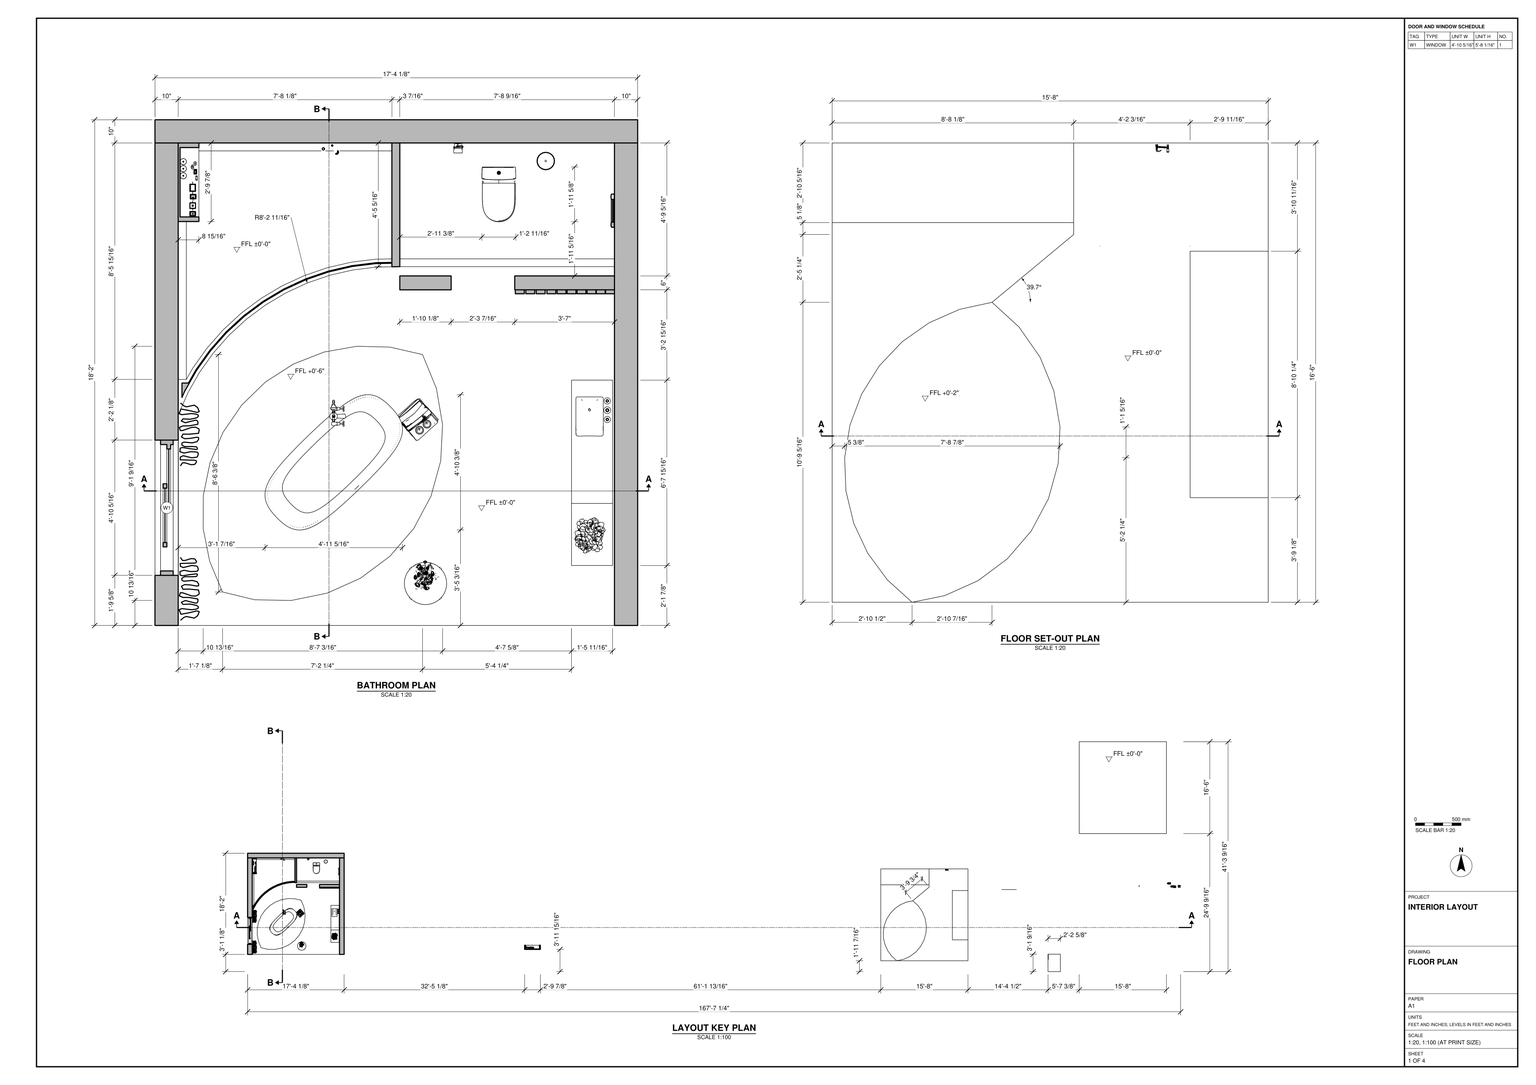
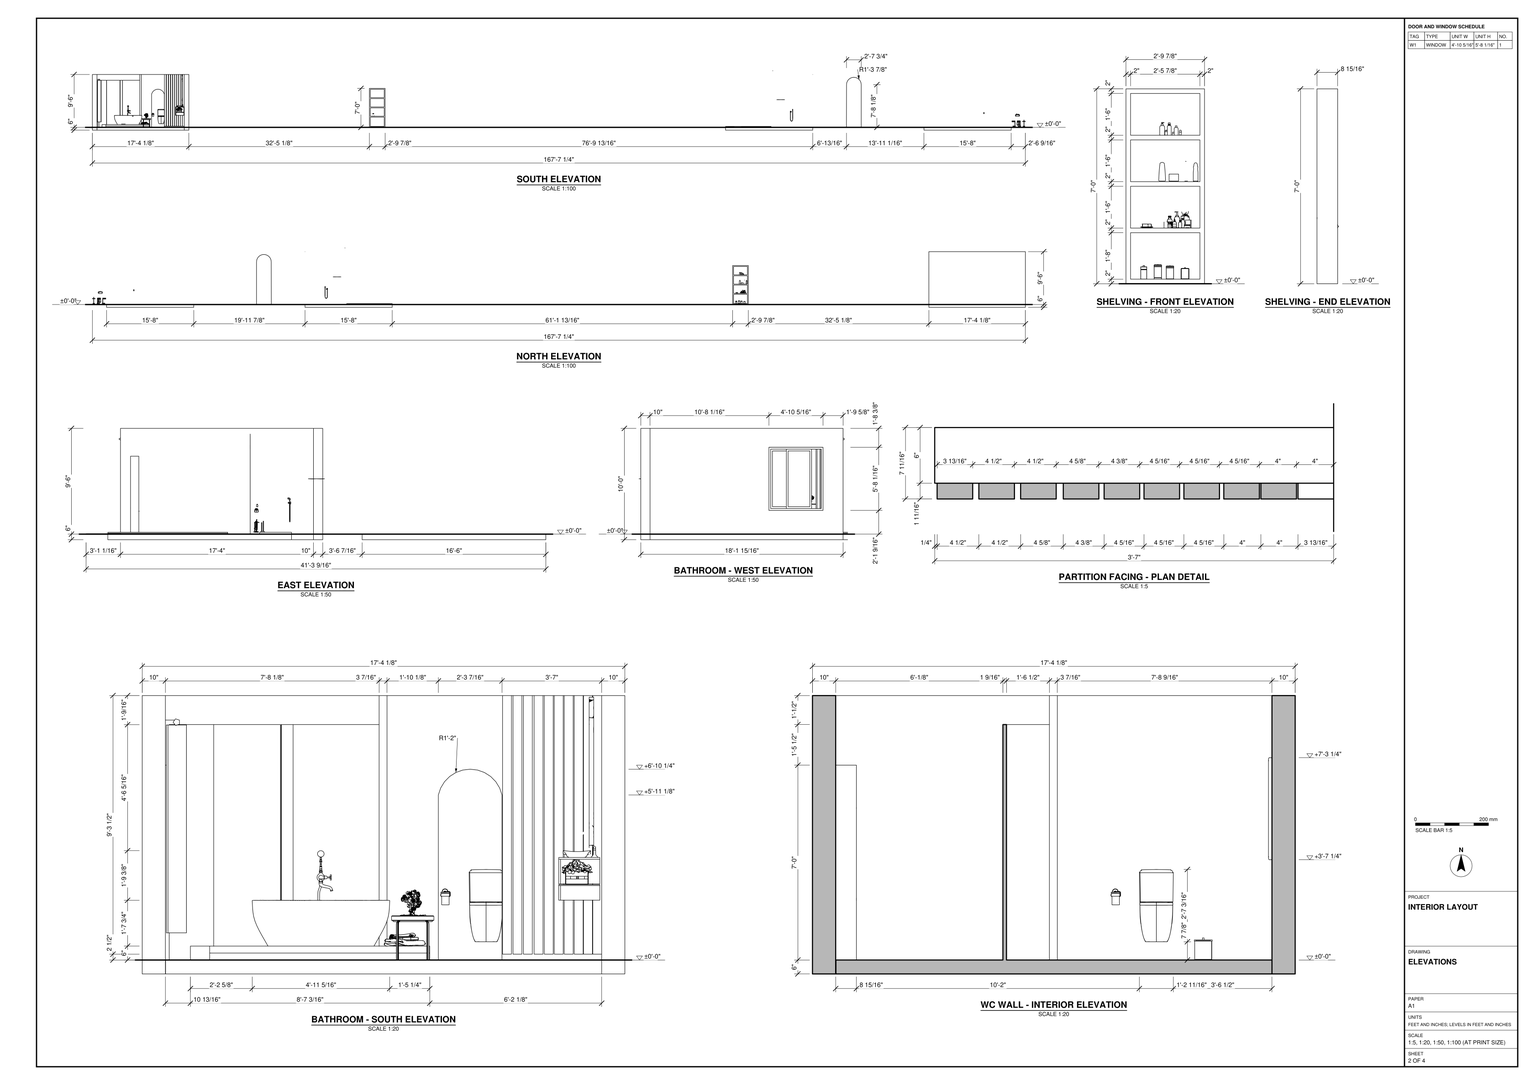
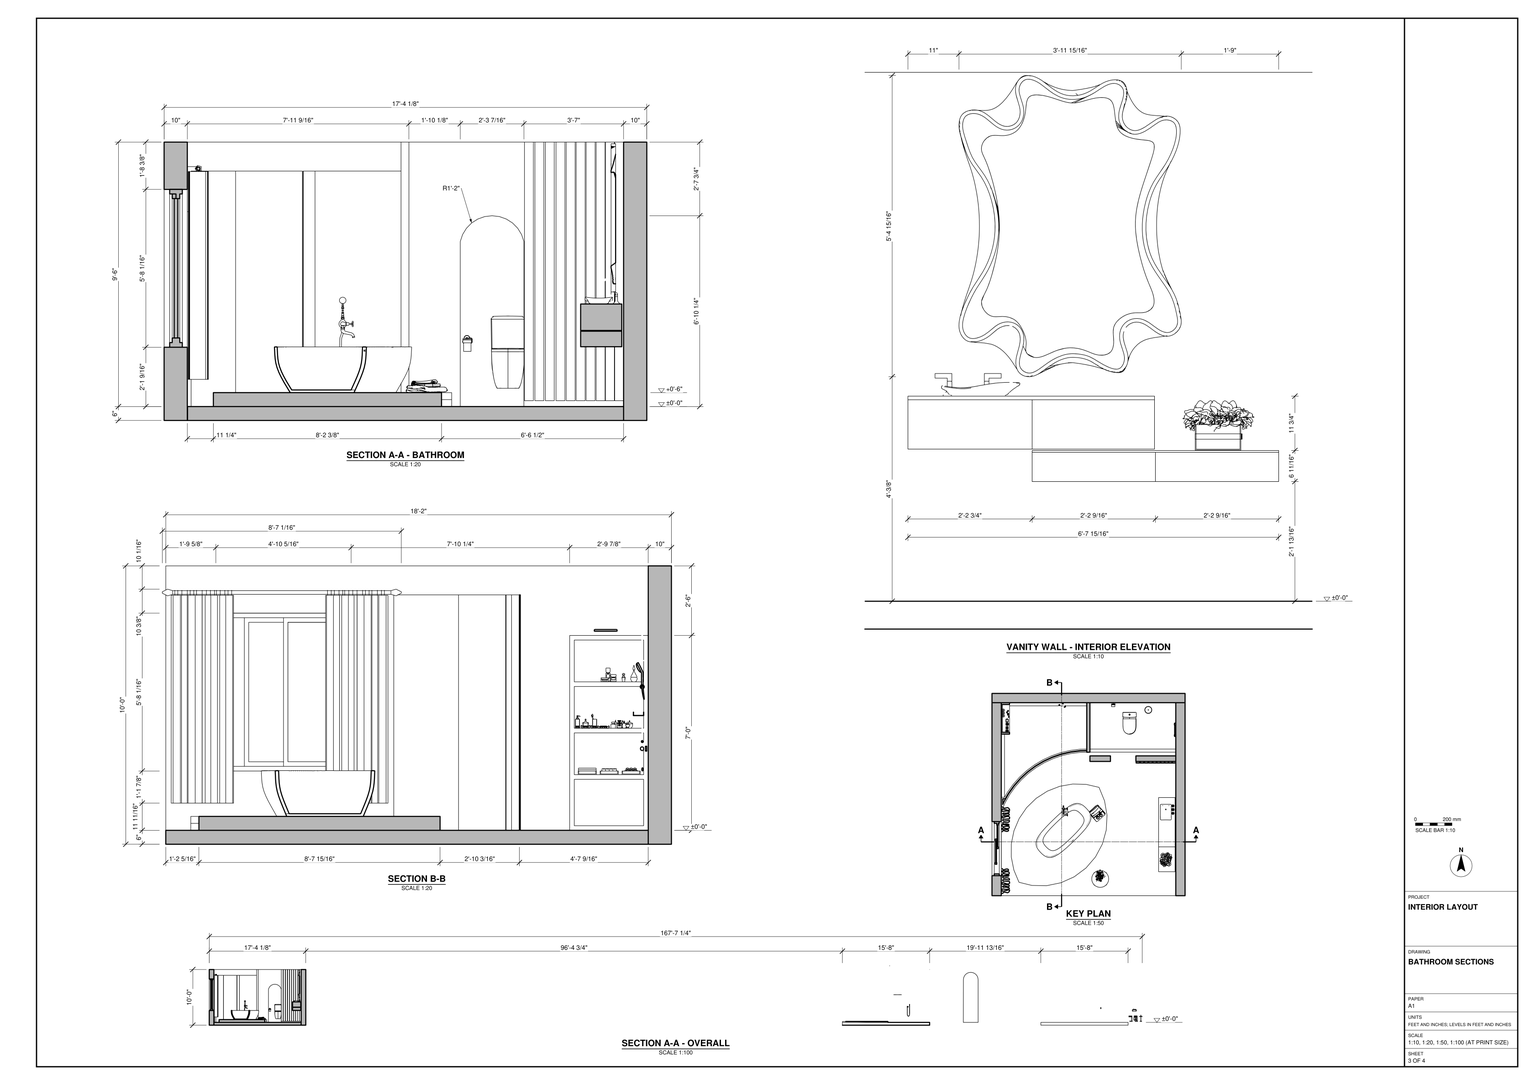
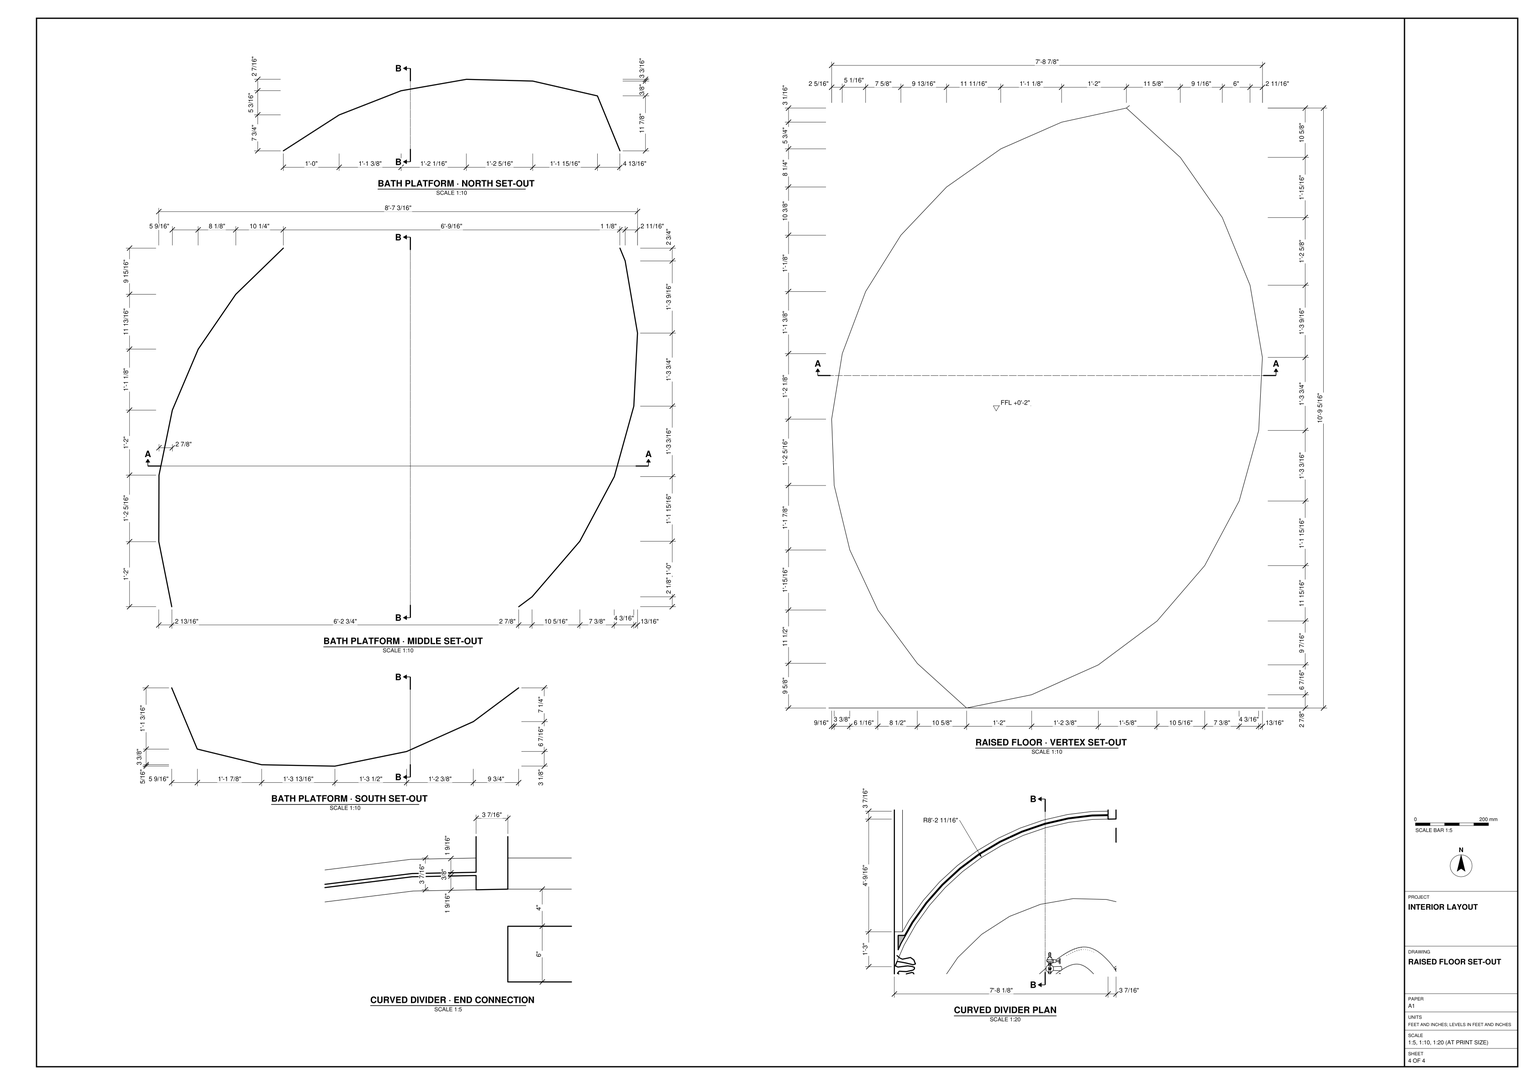
Work in feet and inches in SketchUp using task_files/diagram_01.pdf. Use the layout key plan to position the fitted bathroom at the left and the separate shelving, floor set-out pieces and fittings to its right. Keep the spaces between them as drawn. The complete layout is 167'-7 1/4" along X, 41'-3 9/16" along Y and 10'-0" high. Use ±0'-0" as the single storey datum.

Build the bathroom shell to its own plan dimensions of 17'-4 1/8" by 18'-2", with the floor slab, 10" perimeter walls and internal partitions at their drawn thicknesses. Form the framed west window above its sill. Set the freestanding tub diagonally on the rounded platform, with the tub filler and small table beside it. Follow the curve separating the shower area from the bath, and model the rear toilet compartment with its round-headed opening and adjacent slatted facing.

Use the interior elevations to build the stepped, wall-hung vanity with its basin and mirror, and the open shelving with its horizontal compartments. Reproduce the floor outlines and changes in height shown in the plan and sections, distinguishing the platform in the bathroom from the separate floor set-out. Decor and loose items, including curtains, plants and toiletries, may be any suitable library components.

Keep shell elements and each furniture or joinery piece in separate groups or components, and use components for repeated parts. Save one SketchUp model as output_files/bathroom_interior_and_its_separate_set_out_elements.skp.

# SketchUp Ruby script. Lengths in inches.
U = 1.inch
M = Sketchup.active_model
def pt(a) = Geom::Point3d.new(a.map { |v| v * U })
def face(e, loops, mat)
  f = e.add_face(loops[0].map { |a| pt(a) })
  loops[1..].each { |l| e.add_face(l.map { |a| pt(a) }).erase! }
  f.material = f.back_material = mat if mat
  f
end
# faces: each face lists its corners as indices into pts; further lists are holes
def faces(e, pts, list, mat = nil) = list.each { |f| face(e, (f[0].is_a?(Array) ? f : [f]).map { |l| l.map { |i| pts[i] } }, mat) }
# xy, xz, yz: faces in a plane at the given z, y or x. An outline is a flat list of corners, or four numbers for a rectangle; further outlines are holes
def ring(l) = l.size == 4 ? [[l[0], l[1]], [l[2], l[1]], [l[2], l[3]], [l[0], l[3]]] : l.each_slice(2).to_a
def flat(e, list, mat, &to3) = list.each { |f| face(e, (f[0].is_a?(Array) ? f : [f]).map { |l| ring(l).map { |u, v| to3.(u, v) } }, mat) }
def xy(e, z, list, mat = nil) = flat(e, list, mat) { |x, y| [x, y, z] }
def xz(e, y, list, mat = nil) = flat(e, list, mat) { |x, z| [x, y, z] }
def yz(e, x, list, mat = nil) = flat(e, list, mat) { |y, z| [x, y, z] }
def lines(e, pts, list) = list.each { |a, b| e.add_line(pt(pts[a]), pt(pts[b])) }
# prism: a flat outline (further loops are holes) pulled along v
def prism(e, loops, v, mat = nil)
  f = face(e, loops, mat); d = Geom::Vector3d.new(v.map { |x| x * U })
  f.pushpull(f.normal.samedirection?(d) ? d.length : -d.length)
end
def box(e, o, s, mat = nil) = prism(e, [[o, [o[0] + s[0], o[1], o[2]], [o[0] + s[0], o[1] + s[1], o[2]], [o[0], o[1] + s[1], o[2]]]], [0, 0, s[2]], mat)
def at(x, y, z, deg = 0) = Geom::Transformation.translation(pt([x, y, z])) * Geom::Transformation.rotation(ORIGIN, Z_AXIS, deg.degrees)
def axes(o, x, y, z) = Geom::Transformation.new([*x, 0, *y, 0, *z, 0, *pt(o).to_a, 1])
def part(name) = M.definitions.add(name)
# library, detail: a bought-in or finely detailed component or shape, given as its bounding box
def library(name, o, s) = part(name).tap { |d| box(d.entities, o, s) }
def detail(e, o, s) = box(e.add_group.entities, o, s)
def put(e, d, t, mat = nil) = e.add_instance(d, t).tap { |i| i.material = mat if mat }
def group(e, t, mat = nil) = e.add_group.tap { |g| g.transformation = t; g.material = mat if mat }.entities
root = M.entities
M.materials.add("[Color A01]").color = [255, 204, 204]
M.materials.add("[Color A02]").color = [255, 153, 153]
M.materials.add("[Color B01]").color = [207, 197, 189]
M.materials.add("[Translucent Glass Blue]").color = [100, 149, 237]
M.materials["[Translucent Glass Blue]"].alpha = 0.5
c1 = library("bath+tub",[751.79,-1619.37,0],[68.45,31.82,19.75])
c2 = library("Inodoro ROCA Meridian-N compact",[-14.68,0,0],[14.68,23.62,31.16])
c3 = library("77732 KARE Mirror Drops Oval 14x25cm (Spiegel Drops Oval 14x",[-0.49,-2.625,-0.01],[0.98,5.28,9.78])
c4 = library("Group\#95",[-126.0625,56.51,376.27],[112.05,106.35,108.99])
c5 = library("Group\#96",[-107.16,-137.18,245.54],[76.51,112.05,84.97])
c6 = library("Group\#98",[134.07,-35.59,197.42],[66.93,108.39,101.45])
c7 = library("Group\#99",[44.02,93.6,218.34],[115.22,101.76,105.18])
c8 = library("Group\#100",[-19.56,232.65,283.18],[66.82,42.19,66.65])
c9 = library("Group\#101",[-53.74,7.67,120.98],[106.95,236.74,251.98])
c10 = library("Group\#102",[-49.75,139.84,314.95],[22.11,22.61,22.06])
c11 = library("Group\#103",[-56.625,3.66,294.95],[88.3,152.82,59.14])
c12 = library("Group\#107",[-100.48,19.53,147.87],[113.05,111.28,101.19])
c13 = library("Group\#108",[-54.85,-171.1875,247.55],[90.72,132.3,71.07])
c14 = library("Group\#111",[-161.51,-101.97,314.73],[172.81,108.71,69.27])
c15 = library("Group\#113",[70.77,-125.64,148.84],[102.7,108.07,96.82])
c16 = library("Group\#114",[-28.1,-125.85,106.48],[194.72,128.52,261.01])
c17 = library("Group\#115",[-14.51,-199.73,94.2],[105.22,97.74,77.03])
c18 = library("Group\#116",[-24.89,-182.93,111.64],[113.72,173.94,173.74])
c19 = library("Group\#117",[-7.79,-309.02,238.22],[108.5,93.72,102.44])
c20 = library("Group\#118",[2.57,-271.06,187.04],[93.4,209.89,191.26])
c21 = library("Group\#119",[-21.74,-164.88,146.75],[158.66,158.69,243.45])
c22 = library("Group\#120",[51.13,-202.98,245.86],[103.83,96.91,120.11])
c23 = library("Group\#121",[111.16,-90.29,303.89],[49.95,90,76.18])
c24 = library("Group\#122",[47.44,-177.11,343.1],[125.1,149.08,142.01])
c25 = library("Group\#123",[-80.82,10.33,268.03],[91.87,74,84.35])
c26 = library("Group\#124",[-75.58,-212.0625,396.64],[87.14,69.73,75.82])
c27 = library("Group\#125",[-86.85,-171.15,214.86],[148.39,157.28,240.38])
c28 = library("Group\#126",[-191.98,-250.23,297.57],[97.9,89.36,114.5])
c29 = library("Group\#127",[-192.01,-26.24,304.89],[187.25,107.21,53.21])
c30 = library("Group\#128",[-210.125,-102.4375,276.88],[51.54,90.91,87.28])
c31 = library("Group\#129",[-168.05,-105.3,214.4],[173.05,109.74,165.51])
c32 = library("Group\#130",[-147.09,-43.87,347.03],[63.89,87.81,80.15])
c33 = library("Group\#131",[-110.02,-64.26,144.44],[128.07,118.55,275.77])
c34 = library("Group\#132",[-124.14,3.49,256.66],[120.45,70.64,46.18])
c35 = library("Group\#133",[-118.71,-26.72,138.49],[113,166.64,338.37])
c36 = library("Group\#134",[-159.97,129.63,257.39],[89.36,80.73,106.4])
c37 = library("Group\#135",[-136.13,-14.65,175.64],[147.69,202.17,192.49])
c38 = library("Group\#136",[-5.59,-15.12,374.79],[85.57,86.81,59.51])
c39 = library("Group\#137",[-37.32,-33.18,117.69],[148.47,104.95,286.6])
c40 = library("Group\#138",[-6.61,93.85,461.94],[98.68,62.42,49.38])
c41 = library("Group\#139",[-20.13,5.57,225.44],[155.68,162.88,267.12])
c42 = library("Group\#140",[-80.73,-182.31,261.98],[90.74,132.73,71.97])
c43 = library("Group\#141",[-75.53,-189.01,309.71],[68.94,147.24,88.69])
c44 = library("Group\#142",[-39.42,-209.09,286.91],[66.94,168.34,116.98])
c45 = library("Group\#143",[-81.93,-128.91,211.16],[107.53,90.8,94.63])
c46 = library("Group\#144",[-21.54,14.12,313.18],[84.79,137.02,109.55])
c47 = library("Group\#145",[-45.26,-82.43,273.6875],[73.19,105.45,181.93])
c48 = library("Group\#146",[-10.36,3.03,272.26],[79.07,139.88,53.94])
c49 = library("Group\#147",[24.16,-5.45,296.62],[84.08,128.04,53.21])
c50 = library("Group\#148",[-40.71,1.11,275.78],[91.4,147.63,75.64])
c51 = library("Group\#149",[1.16,-23.73,246.66],[101.27,126.17,86.62])
c52 = library("Group\#150",[-53.8125,-212.33,295.34],[68.49,139.76,73.67])
c53 = library("Group\#151",[-94.36,-157.31,255.2],[101.84,115.08,71.07])
c54 = library("Group\#152",[-39.88,-92.9,113.08],[80.99,54.06,154.09])
c55 = library("Group\#153",[-59.78,14.09,300.39],[101.06,171.37,85.05])
c56 = library("Group\#154",[-39.96,0.65,262.91],[71.32,151.8,74.06])
c57 = library("Group\#155",[-161.17,-232.45,32.75],[152.53,236.06,399.97])
c58 = library("Group\#156",[6.78,-176.96,61.53],[128.84,205.63,400.02])
c59 = library("Group\#157",[-1.6875,-94.42,75.86],[134.92,113.41,305.11])
c60 = library("Group\#158",[-60.84,-159.99,77.97],[92.87,130.98,190.36])
c61 = library("Group\#159",[-62.72,-147.62,57.55],[93.45,86.61,60.22])
c62 = library("Group\#160",[-84.97,-34.6875,78.05],[116.39,151.55,263.18])
c63 = library("Group\#161",[-32.97,-25.89,74.09],[206.79,187.79,274.23])
c64 = library("Group\#162",[-54.58,-83.54,30.99],[209.74,138.81,269.85])
c65 = library("Group\#163",[-44.59,-71.91,-0.375],[108.06,108.06,265.92])
c66 = library("Group\#164",[-41.5,-68.73,2.45],[101.74,101.7,171.82])
c67 = library("Group\#165",[-41.09,-203.71,-2.45],[72.23,68.1,8.96])
c68 = library("Group\#166",[-72.08,-328.41,-0.84],[78.06,90.26,14.33])
c69 = library("Group\#167",[-38.17,-273.34,-0.36],[93.61,85.68,37.86])
c70 = library("Group\#168",[-44.12,-281.8,-0.32],[111.26,106.83,75.57])
c71 = library("Group\#169",[79.9,102.31,0.95],[37.36,48.66,9.9])
c72 = library("Group\#170",[56.48,112.77,1.08],[48.06,25.98,13.89])
c73 = library("Group\#171",[72.44,-147.39,-0.42],[23.31,46.98,9.15])
c74 = library("Group\#172",[210.7,-108.99,0.28],[36.24,50.48,9.9])
c75 = library("Group\#173",[220.9,-124.54,1.08],[13.77,52.12,13.89])
c76 = library("Group\#174",[167.26,-103.49,-0.7],[57.68,26.7,10.44])
c77 = library("Group\#175",[142.48,-79.67,1],[43.05,39.63,15.57])
c78 = library("Group\#176",[248.67,-54.61,-0.08],[36.39,42.46,17.38])
c79 = library("Group\#177",[193.58,-33.21,-1.68],[36.48,42.01,10.95])
c80 = library("Group\#179",[210.09,-29.63,-0.2],[39.11,52.61,14.77])
c81 = library("Group\#180",[-209.51,-88.09,-0.09],[13.54,51.1,15.8])
c82 = library("Group\#181",[-54.86,-136.11,-1.68],[49.86,19.04,10.95])
c83 = library("Group\#183",[-122.87,-196.19,0.47],[48.06,25.97,13.89])
c84 = library("Group\#184",[-150.12,-240.625,-0.4],[11.63,50.1,24.95])
c85 = library("Group\#185",[-116.51,-130.79,0.39],[14.38,57.14,15.57])
c86 = library("Group\#186",[-182.24,-139.72,-0.13],[56.75,40.03,14.2])
c87 = library("Group\#188",[-207.67,30.42,-0.9],[25.63,50.27,12.3])
c88 = library("Group\#189",[-172.77,40.41,-0.51],[21.75,45.25,16.32])
c89 = library("Group\#190",[-180.55,189.74,-0.03],[49.43,32.8,20.41])
c90 = library("Group\#191",[101.2,192.9375,0.85],[30.56,51.07,18.99])
c91 = library("Group\#192",[-229.59,150.48,-0.31],[49.39,18.82,9.67])
c92 = library("Group\#193",[-112.85,170.09,0.27],[33.5,38.18,12.42])
c93 = library("Group\#194",[21.88,30.1,1.13],[19.79,43.29,9.19])
c94 = library("Group\#195",[-79.42,-90.58,1.23],[27.88,43.88,12.3])
c95 = library("Group\#196",[-127.08,-286.71,-0.14],[33.47,50.32,11.84])
c96 = library("Group\#197",[-197.39,99.82,-0.47],[43.11,37.62,15.6])
c97 = library("Group\#199",[-27.41,-124.52,-0.78],[20.93,47.82,9.14])
c98 = library("Group\#200",[26.33,74.99,1.28],[53.38,19.42,14.98])
c99 = library("Group\#201",[10.45,76.82,0.07],[28.28,56.98,13.56])
c100 = library("Group\#202",[-25.11,33.28,1.57],[29.78,42.64,16.1])
c101 = library("Group\#203",[-39.97,68.22,-0.03],[38.63,48.26,26.54])
c102 = library("Group\#204",[164.13,106.84,0.59],[27.38,60.49,14.93])
c103 = library("Group\#205",[-130.15,4.41,-0.48],[48.46,51.92,11.15])
c104 = library("Group\#206",[-189.65,-8.38,0.66],[48.33,31.91,9.88])
c105 = library("Group\#207",[-141.44,-113.37,0.3],[20.53,61.5,14.1])
c106 = library("Group\#208",[-0.86,206.91,0.32],[47.68,39.6,11.54])
c107 = library("Group\#209",[-44.14,156.6,-1.15],[45.04,36.23,10.11])
c108 = library("Group\#210",[20.74,116.14,-1.25],[18.97,49.31,11.1])
c109 = library("Group\#211",[82.73,35.89,0.36],[52.87,25.75,10.37])
c110 = library("Group\#212",[-127.82,-180.79,-0.25],[32.53,51.61,10.43])
c111 = library("Group\#213",[-174.32,-293.63,-0.39],[47.63,19.69,18.01])
c112 = library("Group\#214",[-99.45,-206.66,0.34],[37.36,48.66,9.91])
c113 = library("Group\#215",[-200.03,-84.69,-0.65],[59.14,46.37,12.98])
c114 = library("Group\#216",[-110.43,96.29,-0.82],[45.84,41.98,9.65])
c115 = library("Group\#217",[-81.31,-44.23,0.64],[38.81,47.66,17.39])
c116 = library("Group\#220",[162.0625,4.5,-0.42],[38.34,35.6875,9.15])
c117 = part("flower vase")
p = [[0,0,0],[1,0,0],[1,1,0]]
lines(c117.entities,p,[[0,1],[1,2],[2,0]])
put(c117.entities,c4,at(0,0,0))
put(c117.entities,c5,at(0,0,0))
put(c117.entities,c6,at(0,0,0))
put(c117.entities,c7,at(0,0,0))
put(c117.entities,c8,at(0,0,0))
put(c117.entities,c9,at(0,0,0))
put(c117.entities,c10,at(0,0,0))
put(c117.entities,c11,at(0,0,0))
put(c117.entities,c12,at(0,0,0))
put(c117.entities,c13,at(0,0,0))
put(c117.entities,c14,at(0,0,0))
put(c117.entities,c15,at(0,0,0))
put(c117.entities,c16,at(0,0,0))
put(c117.entities,c17,at(0,0,0))
put(c117.entities,c18,at(0,0,0))
put(c117.entities,c19,at(0,0,0))
put(c117.entities,c20,at(0,0,0))
put(c117.entities,c21,at(0,0,0))
put(c117.entities,c22,at(0,0,0))
put(c117.entities,c23,at(0,0,0))
put(c117.entities,c24,at(0,0,0))
put(c117.entities,c25,at(0,0,0))
put(c117.entities,c26,at(0,0,0))
put(c117.entities,c27,at(0,0,0))
put(c117.entities,c28,at(0,0,0))
put(c117.entities,c29,at(0,0,0))
put(c117.entities,c30,at(0,0,0))
put(c117.entities,c31,at(0,0,0))
put(c117.entities,c32,at(0,0,0))
put(c117.entities,c33,at(0,0,0))
put(c117.entities,c34,at(0,0,0))
put(c117.entities,c35,at(0,0,0))
put(c117.entities,c36,at(0,0,0))
put(c117.entities,c37,at(0,0,0))
put(c117.entities,c38,at(0,0,0))
put(c117.entities,c39,at(0,0,0))
put(c117.entities,c40,at(0,0,0))
put(c117.entities,c41,at(0,0,0))
put(c117.entities,c42,at(0,0,0))
put(c117.entities,c43,at(0,0,0))
put(c117.entities,c44,at(0,0,0))
put(c117.entities,c45,at(0,0,0))
put(c117.entities,c46,at(0,0,0))
put(c117.entities,c47,at(0,0,0))
put(c117.entities,c48,at(0,0,0))
put(c117.entities,c49,at(0,0,0))
put(c117.entities,c50,at(0,0,0))
put(c117.entities,c51,at(0,0,0))
put(c117.entities,c52,at(0,0,0))
put(c117.entities,c53,at(0,0,0))
put(c117.entities,c54,at(0,0,0))
put(c117.entities,c55,at(0,0,0))
put(c117.entities,c56,at(0,0,0))
put(c117.entities,c57,at(0,0,0))
put(c117.entities,c58,at(0,0,0))
put(c117.entities,c59,at(0,0,0))
put(c117.entities,c60,at(0,0,0))
put(c117.entities,c61,at(0,0,0))
put(c117.entities,c62,at(0,0,0))
put(c117.entities,c63,at(0,0,0))
put(c117.entities,c64,at(0,0,0))
put(c117.entities,c65,at(0,0,0))
put(c117.entities,c66,at(0,0,0))
put(c117.entities,c67,at(0,0,0))
put(c117.entities,c68,at(0,0,0))
put(c117.entities,c69,at(0,0,0))
put(c117.entities,c70,at(0,0,0))
put(c117.entities,c71,at(0,0,0))
put(c117.entities,c72,at(0,0,0))
put(c117.entities,c73,at(0,0,0))
put(c117.entities,c74,at(0,0,0))
put(c117.entities,c75,at(0,0,0))
put(c117.entities,c76,at(0,0,0))
put(c117.entities,c77,at(0,0,0))
put(c117.entities,c78,at(0,0,0))
put(c117.entities,c79,at(0,0,0))
g1 = group(c117.entities,at(0,0,0))
detail(g1,[-125.92,-57.19,0],[29.51,42.66,5.27])
put(c117.entities,c80,at(0,0,0))
put(c117.entities,c81,at(0,0,0))
put(c117.entities,c82,at(0,0,0))
g2 = group(c117.entities,at(0,0,0))
detail(g2,[-72.81,-133.6875,-0.86],[7.83,54.32,7.6])
put(c117.entities,c83,at(0,0,0))
put(c117.entities,c84,at(0,0,0))
put(c117.entities,c85,at(0,0,0))
put(c117.entities,c86,at(0,0,0))
g3 = group(c117.entities,at(0,0,0))
detail(g3,[-128.51,132.875,-0.52],[47.95,16.21,8.19])
put(c117.entities,c87,at(0,0,0))
put(c117.entities,c88,at(0,0,0))
put(c117.entities,c89,at(0,0,0))
put(c117.entities,c90,at(0,0,0))
put(c117.entities,c91,at(0,0,0))
put(c117.entities,c92,at(0,0,0))
put(c117.entities,c93,at(0,0,0))
put(c117.entities,c94,at(0,0,0))
put(c117.entities,c95,at(0,0,0))
put(c117.entities,c96,at(0,0,0))
g4 = group(c117.entities,at(0,0,0))
p = [[-27.64,62.67,3.44],[-15.71,68.26,1.48],[-15.66,71.65,0.62],[-21.57,68.97,2.31],[-13.17,69.58,2.55],[-36.26,54.21,1.61],
  [-31.87,53.51,1.99],[-33.2,58.14,1.29],[-31.35,61.65,2.625],[-15.72,67.39,3.15],[-44.8,46.65,5.28],[-47.1,43.13,7.82],
  [-28.86,58.34,3.52],[-29.19,65.03,3.4],[-25.6,67.375,2.31],[-22.51,63.64,4.02],[-26.57,61.08,4.77],[-48.1,43.35,7.41],
  [-48.18,44.3,7.4]]
faces(g4,p,[[0,1,2],[3,0,2],[2,1,4],[5,6,7],[0,7,6],[0,8,7],[0,9,1],[10,6,5],
  [10,11,6],[0,6,12],[13,0,14],[0,3,14],[0,13,8],[0,15,9],[12,16,0],[0,16,15],
  [17,11,10],[10,18,17]])
put(c117.entities,c97,at(0,0,0))
put(c117.entities,c98,at(0,0,0))
put(c117.entities,c99,at(0,0,0))
put(c117.entities,c100,at(0,0,0))
put(c117.entities,c101,at(0,0,0))
put(c117.entities,c102,at(0,0,0))
put(c117.entities,c103,at(0,0,0))
put(c117.entities,c104,at(0,0,0))
put(c117.entities,c105,at(0,0,0))
put(c117.entities,c106,at(0,0,0))
put(c117.entities,c107,at(0,0,0))
put(c117.entities,c108,at(0,0,0))
put(c117.entities,c109,at(0,0,0))
put(c117.entities,c110,at(0,0,0))
put(c117.entities,c111,at(0,0,0))
put(c117.entities,c112,at(0,0,0))
put(c117.entities,c113,at(0,0,0))
put(c117.entities,c114,at(0,0,0))
put(c117.entities,c115,at(0,0,0))
g5 = group(c117.entities,at(0,0,0))
detail(g5,[-41.4,-95.67,-0.33],[35.59,40.51,7.29])
g6 = group(c117.entities,at(0,0,0))
detail(g6,[104.51,196.26,-0.54],[49.32,21.84,6.4])
put(c117.entities,c116,at(0,0,0))
g7 = group(c117.entities,at(0,0,0))
detail(g7,[-145.24,174.98,-1.26],[23.31,40.87,7.36])
g8 = group(c117.entities,at(0,0,0))
detail(g8,[38.73,78.34,-1.01],[51.44,18.24,7.51])
g9 = group(c117.entities,at(0,0,0))
detail(g9,[149.28,-49.43,-0.86],[48.21,27.38,7.6])
c118 = library("skp3DA3",[0,-0.85,0],[1.69,1.7,1.77])
c119 = library("skp31A6",[-6.04,-1.48,35.67],[7.16,7.43,3.03])
c120 = part("Untitled\#1")
xy(c120.entities,0.24,[[159.21,25.41,250.9,90.43]])
# 1 loose lines left out
c121 = library("Window",[11.02,30.31,0],[35.44,3.94,39.37])
c122 = library("Window curtains 2",[0,-81.89,0],[92,82.37,8.12])
c123 = library("Bathroom shower tap",[73.4375,31.53,0],[12.71,23.82,68.1875])
c124 = library("Ambra",[-27.36,0.91,-0.02],[2.82,2.83,5.45])
c125 = library("acessorio 01",[0.27,-0.03,0.08],[14.77,2.81,6.34])
c126 = library("decor 01",[0,0,0],[33.46,7.875,3.66])
c127 = part("Grupo\#26")
prism(c127.entities,[[[6.89,0.59,0],[6.3,0.59,0],[6.3,0.59,8.86],[0,0.59,8.86],[0,0.59,9.45],[6.89,0.59,9.45]]],[0,-0.59,0])
c128 = part("Grupo\#2")
box(c128.entities,[0,0,0],[5.71,3.9375,0.98])
c129 = part("Grupo\#20")
prism(c129.entities,[[[6.89,0.59,0],[6.3,0.59,0],[6.3,0.59,10.43],[0,0.59,10.43],[0,0.59,11.02],[6.89,0.59,11.02]]],[0,-0.59,0])
c130 = part("Grupo\#40")
put(c130.entities,c127,at(0,0.79,0.98))
put(c130.entities,c128,at(1.97,0,0))
put(c130.entities,c129,at(0,2.56,0.98))
c131 = part("Portatoalharosto 01")
put(c131.entities,c130,at(-1.97,0,0))
c132 = library("Portatoalharosto 02",[0,0,0],[6.2,5.1,13.91])
c133 = library("NECESSAIRE",[-4.72,-2.02,0],[9.44,4.04,4.14])
c134 = library("perfume 01",[35.39,9.67,0.08],[11.07,12.43,14.81])
c135 = library("perfume 02",[90.1875,185.875,-17.9],[0.5,0.53,1.3])
c136 = library("Portatoalharosto 03",[0,0,0],[8.23,3.98,12.3125])
c137 = library("decor 03",[-0.35,-0.35,-0.01],[2.79,2.79,7.1])
c138 = library("Group\#83",[0,0,0],[64.94,47.92,1.97])
c139 = library("Group\#224",[0,0,0],[11.43,6.82,41.14])
c140 = part("Difference\#2")
detail(c140.entities,[0,0,0],[92.54,6.01,114])
c141 = library("Group\#76",[0,0,0],[8.9,15.65,16.375])
c142 = library("Group\#75",[0,0,0],[21.4,15.55,54.87])
c143 = library("Group\#74",[0,0,0],[2.19,5.12,12.66])
c144 = library("Group\#73",[0,0,0],[16.48,12.31,18.55])
c145 = library("Group\#72",[0,0,0],[18.48,12.82,12.92])
c146 = library("Group\#71",[0,0,0],[27.43,40.05,11.5])
c147 = library("Group\#70",[0,0,0],[4.72,20.47,20.47])
c148 = library("Group\#69",[0,0,0],[9.25,9.25,9.84])
c149 = library("Group\#67",[0,0,0],[8.86,8.73,5.05])
c150 = library("Group\#66",[0,0,0],[9.25,9.25,9.84])
c151 = library("Group\#65",[0,0,0],[8.35,91.71,210.87])
c152 = library("Group\#77",[0,0,0],[7.875,7.875,11.8125])
c153 = library("Group\#78",[0,0,0],[8.25,8.25,1.97])
c154 = library("Grupo\#10",[0,0,0],[10.67,10.39,17.07])
c155 = part("Difference")
prism(c155.entities,[[[10,0,0],[10,208,0],[10,208,120],[10,0,120]],[[10,21.6,31.57],[10,21.6,99.6],[10,79.91,99.6],[10,79.91,31.57]]],[-10,0,0])
c156 = library("Group\#249",[0,0,0],[92.85,129.3125,6])
c157 = library("Group\#228",[-3.29,0,0],[22.24,79.92,29.79])
c158 = library("Group\#251",[0,0,0],[33.87,8.9375,84])
c159 = library("Group\#252",[0,0,0],[15.88,12.56,5.72])
c160 = library("Group\#253",[0,0,0],[33.87,9.36,84])
xy(root,-6,[[1364.86,23.42,1552.86,221.42],[10.1,37.1,198.1,245.1]])
xy(root,0,[[1399.34,23.42,1552.86,23.42,1552.86,68.51,1519.19,68.51,1519.19,174.75,1552.86,174.75,1552.86,221.42,1469,221.42,1469,181.95,1462.89,176.875,1462.88,176.87,1462.86,176.85,1433.8,152.73,1445.43,142.07,1454.46,129.14,1460.45,114.54,1463.11,98.99,1462.3125,83.24,1458.1,68.03,1450.67,54.11,1440.39,42.15,1427.74,32.72,1413.34,26.27],[1519.19,68.51,1552.86,174.75],[10.1,128.0625,14.2,137.41,19.24,146.28,25.17,154.58,31.92,162.22,39.43,169.13,47.61,175.23,56.38,180.44,65.64,184.73,75.29,188.04,85.23,190.33,95.36,191.58,102.14,191.72,102.14,193.25,95.25,193.12,84.97,191.84,74.87,189.52,65.07,186.16,60.02,183.82,59.61,183.63,55.66,181.81,46.76,176.51,38.45,170.32,30.82,163.3,23.96,155.54,17.94,147.1,12.82,138.1,11.64,135.39,11.64,141.6,14.42,141.6,17.65,147.29,23.69,155.75,30.58,163.54,38.23,170.58,46.57,176.8,55.5,182.11,59.46,183.95,59.875,184.14,64.9375,186.48,74.77,189.85,84.91,192.1875,95.22,193.46,102.14,193.6,102.14,195.14,95.11,195,84.64,193.7,74.35,191.33,64.36,187.91,54.78,183.48,45.71,178.08,37.25,171.77,29.48,164.62,22.49,156.71,16.35,148.12,13.52,143.14,10.1,143.14],[10.1,143.14,13.52,143.14,13.52,241.67,102.14,241.67,102.14,245.1,10.1,245.1],[13.52,143.14,16.35,148.12,22.49,156.71,29.48,164.62,37.25,171.77,45.71,178.08,54.78,183.48,64.36,187.91,74.35,191.33,84.64,193.7,95.11,195,102.14,195.14,102.14,241.67,13.52,241.67],
  [1462.86,176.85,1462.88,176.87,1462.86,176.875],[1462.88,176.87,1462.89,176.875,1462.86,176.875],[59.61,183.63,60.02,183.82,59.875,184.14,59.46,183.95],[105.56,191.78,198.1,195.14],[105.56,195.14,198.1,245.1]])
xy(root,0,[[10.1,37.1,198.1,37.1,198.1,191.78,105.56,191.78,102.14,191.72,95.36,191.58,85.23,190.33,75.29,188.04,65.64,184.73,56.38,180.44,47.61,175.23,39.43,169.13,31.92,162.22,25.17,154.58,19.24,146.28,14.2,137.41,10.1,128.0625]],"[Color B01]")
xy(root,2,[[1399.34,23.42,1413.34,26.27,1427.74,32.72,1440.39,42.15,1450.67,54.11,1458.1,68.03,1462.3125,83.24,1463.11,98.99,1460.45,114.54,1454.46,129.14,1445.43,142.07,1433.8,152.73,1419.82,149.6875,1406.72,143.9375,1395.02,135.71,1385.18,125.32,1377.58,113.2,1372.54,99.81,1370.25,85.68,1370.8,71.39,1374.17,57.48,1380.23,44.52,1388.73,33.02],[1462.86,176.85,1462.88,176.87,1462.86,176.875]])
xy(root,101.5,[[11.64,135.39,12.82,138.1,17.94,147.1,23.96,155.54,30.82,163.3,30.58,163.54,23.69,155.75,17.65,147.29,14.42,141.6,11.64,141.6],[30.82,163.3,38.45,170.32,46.76,176.51,55.66,181.81,59.61,183.63,59.46,183.95,55.5,182.11,46.57,176.8,38.23,170.58,30.58,163.54],[60.02,183.82,65.07,186.16,74.87,189.52,84.97,191.84,95.25,193.12,102.14,193.25,102.14,193.6,95.22,193.46,84.91,192.1875,74.77,189.85,64.9375,186.48,59.875,184.14]])
xy(root,114,[[102.14,191.72,105.56,191.78,105.56,245.1,102.14,245.1]])
xz(root,23.42,[[1364.86,-6,1552.86,-6,1552.86,0,1399.34,0,1399.34,2,1364.86,2]])
xz(root,37.1,[[10.1,-6,198.1,0]])
xz(root,141.6,[[11.64,0,14.42,101.5]])
xz(root,217.61,[[1509.51,37.91,1509.52,37.91,1509.51,37.93]])
xz(root,219.74,[[1509.5625,33.14,1509.63,33.16,1509.63,33.28,1509.5625,33.26]])
xz(root,221.42,[[1364.86,-6,1552.86,0],[1364.86,0,1364.86,2,1469,0]])
xz(root,245.1,[[10.1,-6,10.1,0,102.14,0,102.14,114,105.56,114,105.56,0,198.1,0,198.1,-6]])
yz(root,10.1,[[37.1,-6,245.1,0]])
yz(root,11.64,[[135.39,0,141.6,101.5]])
yz(root,102.14,[[191.72,0,193.25,114],[193.6,0,195.14,114],[195.14,0,241.67,114],[241.67,0,245.1,114],[193.25,101.5,193.6,114]])
yz(root,105.56,[[191.78,0,195.14,114],[195.14,0,245.1,114]])
yz(root,198.1,[[37.1,-6,245.1,0]])
yz(root,1509.47,[[219.4375,33.22,219.54,33.32]])
yz(root,1509.58,[[220.08,37.625,219.61,38.49,219.75,38.32,219.87,38.13,219.98,37.95,220.08,37.75,220.14,37.67]])
yz(root,1509.6,[[220.08,37.625,220.14,37.67,220.08,37.75,219.98,37.95,219.87,38.13,219.75,38.32,219.61,38.49]])
yz(root,1552.86,[[23.42,-6,221.42,0]])
# 752 loose lines left out
p = [[1413.34,26.27,0],[1413.34,26.27,1],[1399.34,23.42,1],[1399.34,23.42,0],[1427.74,32.72,0],[1427.74,32.72,1],
  [1440.39,42.15,0],[1440.39,42.15,1],[1450.67,54.11,0],[1450.67,54.11,1],[1458.1,68.03,0],[1458.1,68.03,1],
  [1462.3125,83.24,0],[1462.3125,83.24,1],[1463.11,98.99,0],[1463.11,98.99,1],[1460.45,114.54,0],[1460.45,114.54,1],
  [1454.46,129.14,0],[1454.46,129.14,1],[1445.43,142.07,0],[1445.43,142.07,1],[11.64,135.39,0],[12.82,138.1,0],
  [12.82,138.1,101.5],[11.64,135.39,101.5],[17.94,147.1,0],[17.94,147.1,101.5],[17.65,147.29,0],[14.42,141.6,0],
  [14.42,141.6,101.5],[17.65,147.29,101.5],[1433.8,152.73,0],[1433.8,152.73,1],[23.96,155.54,0],[23.96,155.54,101.5],
  [23.69,155.75,0],[23.69,155.75,101.5],[30.82,163.3,0],[30.82,163.3,101.5],[30.58,163.54,0],[30.58,163.54,101.5],
  [38.45,170.32,0],[38.45,170.32,101.5],[38.23,170.58,0],[38.23,170.58,101.5],[46.76,176.51,0],[46.76,176.51,101.5],
  [46.57,176.8,0],[46.57,176.8,101.5],[55.66,181.81,0],[55.66,181.81,101.5],[55.5,182.11,0],[55.5,182.11,101.5],
  [59.61,183.63,0],[59.61,183.63,101.5],[59.46,183.95,0],[59.46,183.95,101.5],[59.875,184.14,0],[60.02,183.82,0],
  [60.02,183.82,101.5],[59.875,184.14,101.5],[65.07,186.16,0],[65.07,186.16,101.5],[64.9375,186.48,0],[64.9375,186.48,101.5],
  [74.87,189.52,0],[74.87,189.52,101.5],[74.77,189.85,0],[74.77,189.85,101.5],[84.97,191.84,0],[84.97,191.84,101.5],
  [84.91,192.1875,0],[84.91,192.1875,101.5],[102.14,191.72,0],[105.56,191.78,0],[105.56,191.78,114],[102.14,191.72,114],
  [95.25,193.12,0],[95.25,193.12,101.5],[95.22,193.46,0],[95.22,193.46,101.5],[102.14,193.25,0],[102.14,193.25,101.5],
  [102.14,193.6,0],[102.14,193.6,101.5],[1399.34,23.42,2],[1413.34,26.27,2],[1427.74,32.72,2],[1440.39,42.15,2],
  [1450.67,54.11,2],[1458.1,68.03,2],[1462.3125,83.24,2],[1463.11,98.99,2],[1460.45,114.54,2],[1454.46,129.14,2],
  [1445.43,142.07,2],[1433.8,152.73,2],[1509.52,219.24,33.25],[1509.52,219.24,33.13],[1509.46,219.32,33.11],[1509.46,219.32,33.23],
  [1509.59,219.2,33.27],[1509.59,219.2,33.15],[1509.66,219.23,33.29],[1509.66,219.23,33.17],[1509.43,219.45,33.1],[1509.43,219.45,33.22],
  [1509.45,219.58,33.11],[1509.45,219.58,33.23],[1509.49,219.68,33.12],[1509.49,219.68,33.24],[1509.5625,219.74,33.14],[1509.5625,219.74,33.26],
  [1509.72,219.31,33.31],[1509.72,219.31,33.1875],[1509.49,219.34,33.33],[1509.49,219.34,33.23],[1509.47,219.4375,33.22],[1509.47,219.4375,33.32],
  [1509.54,219.28,33.34],[1509.54,219.28,33.25],[1509.75,219.4375,33.32],[1509.75,219.4375,33.2],[1509.74,219.56,33.3125],[1509.74,219.56,33.19],
  [1509.47,219.54,33.32],[1509.47,219.54,33.22],[1509.51,219.63,33.24],[1509.51,219.63,33.33],[1509.56,219.68,33.26],[1509.56,219.68,33.35],
  [1509.7,219.67,33.3],[1509.7,219.67,33.18],[1509.63,219.74,33.28],[1509.63,219.74,33.16],[1509.6,219.26,33.36],[1509.6,219.26,33.27],
  [1509.65,219.29,33.38],[1509.65,219.29,33.29],[1509.7,219.36,33.39],[1509.7,219.36,33.31],[1509.72,219.46,33.4],[1509.72,219.46,33.32],
  [1509.71,219.56,33.39],[1509.71,219.56,33.3125],[1509.61,219.69,33.36],[1509.61,219.6875,33.28],[1509.67,219.64,33.3],[1509.67,219.64,33.38],
  [1509.58,220.08,37.625],[1509.6,220.08,37.625],[1509.6,219.61,38.49],[1509.58,219.61,38.49],[1509.6,220.14,37.67],[1509.58,220.14,37.67],
  [1509.58,220.08,37.75],[1509.58,219.98,37.95],[1509.6,219.98,37.95],[1509.6,220.08,37.75],[1509.58,219.87,38.13],[1509.6,219.87,38.13],
  [1509.58,219.75,38.32],[1509.6,219.75,38.32]]
faces(root,p,[[0,1,2,3],[4,5,1,0],[6,7,5,4],[8,9,7,6],[10,11,9,8],[12,13,11,10],[14,15,13,12],[16,17,15,14],
  [18,19,17,16],[20,21,19,18],[32,33,21,20],[54,56,57,55],[58,59,60,61],[74,75,76,77],[86,2,1,87],[87,1,5,88],
  [88,5,7,89],[89,7,9,90],[90,9,11,91],[91,11,13,92],[92,13,15,93],[93,15,17,94],[94,17,19,95],[95,19,21,96],
  [96,21,33,97],[98,99,100,101],[102,103,99,98],[104,105,103,102],[101,100,106,107],[107,106,108,109],[109,108,110,111],[111,110,112,113],
  [114,115,105,104],[116,117,118,119],[120,121,117,116],[122,123,115,114],[124,125,123,122],[126,127,128,129],[129,128,130,131],[132,133,125,124],
  [134,135,133,132],[136,137,121,120],[138,139,137,136],[140,141,139,138],[142,143,141,140],[144,145,143,142],[146,147,148,149],[149,148,145,144],
  [131,130,147,146],[150,151,152,153],[154,151,150,155],[156,157,158,159],[155,156,159,154],[160,161,158,157],[162,163,161,160],[152,163,162,153]])
faces(root,p,[[22,23,24,25],[23,26,27,24],[28,29,30,31],[26,34,35,27],[36,28,31,37],[34,38,39,35],[40,36,37,41],[38,42,43,39],
  [44,40,41,45],[42,46,47,43],[48,44,45,49],[46,50,51,47],[52,48,49,53],[50,54,55,51],[56,52,53,57],[59,62,63,60],
  [64,58,61,65],[62,66,67,63],[68,64,65,69],[66,70,71,67],[72,68,69,73],[70,78,79,71],[80,72,73,81],[78,82,83,79],
  [84,80,81,85]],"[Translucent Glass Blue]")
detail(root,[1509.46,220.11,37.76],[0.27,0.08,0.06])
detail(root,[1509.46,220.16,37.67],[0.27,0.08,0.06])
detail(root,[1509.46,220.21,37.58],[0.27,0.08,0.06])
detail(root,[1509.5,219.82,33.94],[0.18,0.08,0.3])
detail(root,[1509.5,219.82,33.14],[0.18,0.08,0.28])
detail(root,[1509.85,217.51,38.33],[0.01,0.04,0.05])
detail(root,[1509.83,217.54,38.21],[0.02,0.04,0.04])
detail(root,[1509.67,217.61,37.93],[0.01,0.04,0.03])
detail(root,[1509.51,217.41,38.75],[0.01,0.04,0.04])
detail(root,[1509.58,217.45,38.6],[0.02,0.04,0.02])
put(root,c1,at(1756.74,-498.88,6,-135.962))
put(root,c2,at(140.91,234.72,7.87,-180))
put(root,c3,axes([197.34,215.79,43.26],[-1.53846,0,0],[0,4.5,0],[0,0,4.5]))
put(root,c117,axes([116.17,59.05,19.13],[0.02183,0,0],[0,0.02183,0],[0,0,0.02183]))
put(root,c118,axes([107.51,55.22,0],[10.77,0,0],[0,10.77,0],[0,0,10.77]))
put(root,c119,axes([119.39,125.93,-59.99],[1.37913,1.23309,0],[-1.23309,1.37913,0],[0,0,1.85]))
put(root,c120,axes([1762.43,-65.28,0.4],[0,0.41,0],[-0.41,0,0],[0,0,0.41]))
put(root,c121,axes([-39.56,135.14,25.57],[0,-1.64558,0],[1.384,0,0],[0,0,1.72939]))
put(root,c122,axes([10,35.6,103.43],[0,1.12,0],[0,0,1.12],[1.12,0,0]),"[Color A02]")
put(root,c123,at(-6.3,189.75,24.07))
put(root,c124,axes([1935.35,183.22,29.52],[0.52,0,0],[0,0.52,0],[0,0,0.52]))
put(root,c125,at(14.96,228.62,43.68,-90))
put(root,c126,axes([12.64,241.66,23.99],[0,-0.8,0],[0.8,0,0],[0,0,0.8]))
put(root,c131,at(1984.17,188.24,1.97))
put(root,c132,at(2005.08,181.36,1.97))
put(root,c133,at(1994.22,183.62,23.62,-180))
put(root,c134,axes([24.65,203.81,63.98],[0,0.59072,0],[-0.59072,0,0],[0,0,0.40169]))
put(root,c135,axes([1045.04,-260.53,162.87],[0,5.5224,0],[-5.5224,0,0],[0,0,5.5224]))
put(root,c136,at(1992.97,180.81,1.97))
put(root,c137,axes([16.97,233.92,64.04],[0,0.52,0],[-0.52,0,0],[0,0,0.52]))
g10 = group(root,at(1792.7,297.54,-6))
box(g10,[0,0,0],[188,198,6])
put(root,c138,axes([194.66,131.875,113.33],[0,0,-1],[0,-1,0],[-1,0,0]))
put(root,c139,at(82.2,122.88,6,90))
g11 = group(root,at(198.1,37.1,-6))
xy(g11,0,[[0,0,10,208]])
xy(g11,120,[[0,0,10,208]])
xz(g11,0,[[0,0,10,120]])
xz(g11,208,[[0,0,10,120]])
yz(g11,0,[[0,0,208,120]],"[Color A01]")
yz(g11,10,[[0,0,208,120]])
put(root,c140,at(105.56,181.78,0),"[Color A01]")
put(root,c141,axes([1509.16,218.19,37.65],[0,-0.09517,0],[0.05567,0,0],[0,0,0.09517]))
put(root,c142,axes([1509.16,219.9,34.03],[0,-0.09517,0],[0.05567,0,0],[0,0,0.09517]))
put(root,c143,axes([1509.45,219.14,35.625],[0,-0.09517,0],[0.05567,0,0],[0,0,0.09517]))
put(root,c144,axes([1509.25,220.36,37.42],[0,-0.09517,0],[0.05567,0,0],[0,0,0.09517]))
put(root,c145,axes([1509.24,220.7,33.0625],[0,-0.09517,0],[0.05567,0,0],[0,0,0.09517]))
put(root,c146,axes([1504.49,220.25,33.2],[0,-0.09517,0],[0.05567,0,0],[0,0,0.09517]))
put(root,c147,axes([1504.24,220.7,32.77],[0,-0.09517,0],[0.05567,0,0],[0,0,0.09517]))
put(root,c148,axes([1504.55,220.17,32.04],[0,-0.09517,0],[0.05567,0,0],[0,0,0.09517]))
put(root,c149,axes([1504.5625,220.15,32.98],[0,-0.09517,0],[0.05567,0,0],[0,0,0.09517]))
put(root,c150,axes([1509.33,219.91,33.1],[0,-0.09517,0],[0.05567,0,0],[0,0,0.09517]))
put(root,c151,axes([1504.65,220,13.13],[0,-0.09517,0],[0.05567,0,0],[0,0,0.09517]))
put(root,c152,axes([164.8,233.64,0],[0.9353,0,0],[0,0.9353,0],[0,0,0.71083]))
put(root,c153,axes([164.62,233.45,8.12],[0.9353,0,0],[0,0.9353,0],[0,0,0.71083]))
put(root,c154,axes([128.67,245.1,23.78],[0,-0.40551,0],[0.40551,0,0],[0,0,0.40551]))
g12 = group(root,at(20.1,245.1,-6),"[Color A01]")
box(g12,[-20.1,0,0],[208.1,10,120])
put(root,c155,at(0,37.1,-6),"[Color A01]")
put(root,c156,at(2.78,63.94,0,-25.2),"[Color B01]")
put(root,c157,at(179.58,62.95,25.8))
g13 = group(root,at(194.27,180.09,2.52),"[Color A02]")
box(g13,[0,0,0],[3.83,1.7,111.48])
put(root,c158,at(18.9375,211.23,0,90))
put(root,c159,axes([18.28,228.99,44],[0,0.5916,0],[-0.5916,0,0],[0,0,0.5916]))
put(root,c160,at(597.2,47.91,0))
g14 = group(root,at(155.37,180.09,2.52),"[Color A02]")
box(g14,[0,0,0],[3.83,1.7,111.48])
g15 = group(root,at(159.87,180.09,2.52),"[Color A02]")
box(g15,[0,0,0],[3.83,1.7,111.48])
g16 = group(root,at(164.37,180.09,2.52),"[Color A02]")
box(g16,[0,0,0],[3.83,1.7,111.48])
g17 = group(root,at(168.97,180.09,2.52),"[Color A02]")
box(g17,[0,0,0],[3.83,1.7,111.48])
g18 = group(root,at(173.37,180.09,2.52),"[Color A02]")
box(g18,[0,0,0],[3.83,1.7,111.48])
g19 = group(root,at(177.67,180.09,2.52),"[Color A02]")
box(g19,[0,0,0],[3.83,1.7,111.48])
g20 = group(root,at(181.97,180.09,2.52),"[Color A02]")
box(g20,[0,0,0],[3.83,1.7,111.48])
g21 = group(root,at(186.27,180.09,2.52),"[Color A02]")
box(g21,[0,0,0],[3.83,1.7,111.48])
g22 = group(root,at(190.27,180.09,2.52),"[Color A02]")
box(g22,[0,0,0],[3.83,1.7,111.48])
